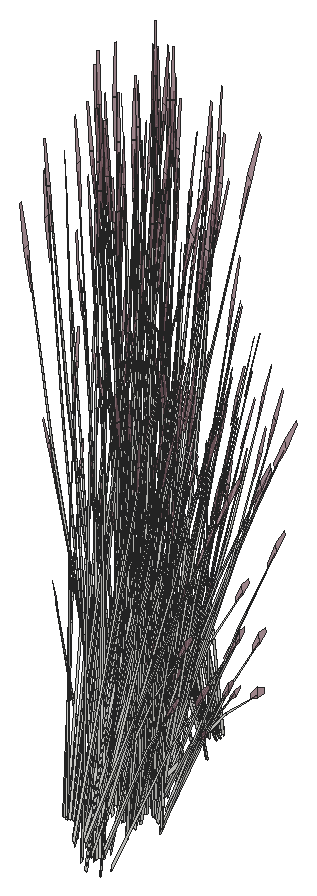
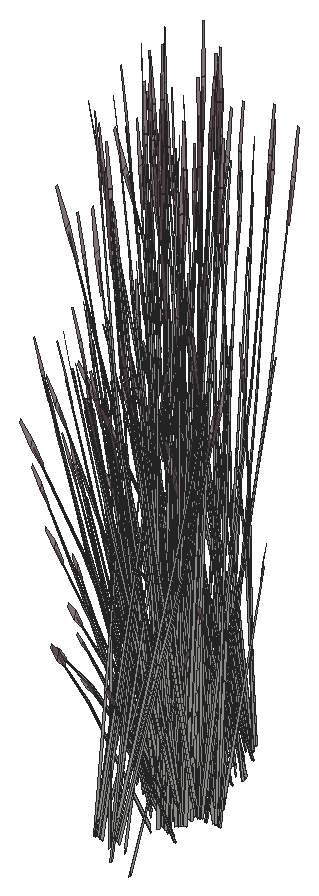
# SketchUp Ruby script. Lengths in inches.
U = 1.inch
M = Sketchup.active_model
def pt(a) = Geom::Point3d.new(a.map { |v| v * U })
def face(e, loops, mat)
  f = e.add_face(loops[0].map { |a| pt(a) })
  loops[1..].each { |l| e.add_face(l.map { |a| pt(a) }).erase! }
  f.material = f.back_material = mat if mat
  f
end
# faces: each face lists its corners as indices into pts; further lists are holes
def faces(e, pts, list, mat = nil) = list.each { |f| face(e, (f[0].is_a?(Array) ? f : [f]).map { |l| l.map { |i| pts[i] } }, mat) }
# xy, xz, yz: faces in a plane at the given z, y or x. An outline is a flat list of corners, or four numbers for a rectangle; further outlines are holes
def ring(l) = l.size == 4 ? [[l[0], l[1]], [l[2], l[1]], [l[2], l[3]], [l[0], l[3]]] : l.each_slice(2).to_a
def flat(e, list, mat, &to3) = list.each { |f| face(e, (f[0].is_a?(Array) ? f : [f]).map { |l| ring(l).map { |u, v| to3.(u, v) } }, mat) }
def xy(e, z, list, mat = nil) = flat(e, list, mat) { |x, y| [x, y, z] }
def xz(e, y, list, mat = nil) = flat(e, list, mat) { |x, z| [x, y, z] }
def yz(e, x, list, mat = nil) = flat(e, list, mat) { |y, z| [x, y, z] }
def lines(e, pts, list) = list.each { |a, b| e.add_line(pt(pts[a]), pt(pts[b])) }
# prism: a flat outline (further loops are holes) pulled along v
def prism(e, loops, v, mat = nil)
  f = face(e, loops, mat); d = Geom::Vector3d.new(v.map { |x| x * U })
  f.pushpull(f.normal.samedirection?(d) ? d.length : -d.length)
end
def box(e, o, s, mat = nil) = prism(e, [[o, [o[0] + s[0], o[1], o[2]], [o[0] + s[0], o[1] + s[1], o[2]], [o[0], o[1] + s[1], o[2]]]], [0, 0, s[2]], mat)
def at(x, y, z, deg = 0) = Geom::Transformation.translation(pt([x, y, z])) * Geom::Transformation.rotation(ORIGIN, Z_AXIS, deg.degrees)
def axes(o, x, y, z) = Geom::Transformation.new([*x, 0, *y, 0, *z, 0, *pt(o).to_a, 1])
def part(name) = M.definitions.add(name)
# library, detail: a bought-in or finely detailed component or shape, given as its bounding box
def library(name, o, s) = part(name).tap { |d| box(d.entities, o, s) }
def detail(e, o, s) = box(e.add_group.entities, o, s)
def put(e, d, t, mat = nil) = e.add_instance(d, t).tap { |i| i.material = mat if mat }
def group(e, t, mat = nil) = e.add_group.tap { |g| g.transformation = t; g.material = mat if mat }.entities
root = M.entities
M.materials.add("LightPink_Translucent").color = [144, 107, 117]
M.materials["LightPink_Translucent"].alpha = 0.75
c1 = part("blade")
p = [[2.15,0.21,22],[0,0.17,0],[0.09,0.45,0],[2.18,0.31,22],[2.29,0.31,22],[0.38,0.45,0],
  [2.48,0.24,33],[2.49,0.24,33],[2.48,0.22,33]]
faces(c1.entities,p,[[0,1,2,3],[4,5,2,3],[6,3,4,7],[8,0,3,6]])
c2 = part("seeds")
p = [[0.3,-0.1,1.38],[-0.01,-0.03,1.59],[-0.01,-0.03,0.03],[0.14,-0.07,-0.07],[0.29,-0.03,3],[0.15,0.01,3.11]]
faces(c2.entities,p,[[0,1,2,3],[1,0,4,5]],"LightPink_Translucent")
c3 = part("blade with seeds")
put(c3.entities,c1,at(0,0,0))
put(c3.entities,c2,axes([2.4,0.25,30.99],[1.5799,-0.05474,1.17369],[-0.12525,1.92788,0.29478],[-0.07173,-0.02425,1.56792]))
put(root,c3,axes([410.79,313.69,-7.3],[-0.07899,-0.43781,0.32977],[0.45153,-0.11561,-0.42575],[0.12128,0.12546,0.81462]))
put(root,c3,axes([410.94,313.53,-9.83],[0.64025,0.17667,0.2864],[-0.16018,0.63149,-0.33981],[-0.10597,0.07904,1.53541]))
put(root,c3,axes([410.89,313.96,-10.12],[-0.47863,0.27177,-0.46235],[-0.28609,-0.48733,0],[-0.10901,0.0619,1.46668]))
put(root,c3,axes([412.48,312.35,-10.12],[0,0.54355,-0.46235],[-0.57217,0,0],[0,0.1238,1.46668]))
put(root,c3,axes([411.05,312.41,-8.39],[-0.18996,-0.09365,1.59586],[0.39312,-0.39287,0.12904],[0.24502,0.17723,0.68222]))
put(root,c3,axes([411.09,311.18,-7.83],[-0.44191,-0.28242,1.28769],[0.46662,-0.43971,0.5556],[0.14258,0.26499,1.24467]))
put(root,c3,axes([407.39,319.84,-10.05],[-0.21003,-0.55738,-0.65031],[0.60499,-0.20074,-0.17068],[-0.02321,-0.18874,1.43544]))
put(root,c3,axes([410.2,318.14,-10.61],[-0.07655,-0.04282,1.6421],[-0.19662,-0.47839,-0.25086],[0.13264,-0.12982,0.2797]))
put(root,c3,axes([411.76,313.47,-9.42],[-0.28795,-0.15629,1.06958],[0.37181,-0.1588,0.78586],[0.10029,0.13452,0.23558]))
put(root,c3,axes([410.75,313.92,-7.3125],[0.30474,-0.46525,-0.11324],[0.44133,0.26804,-0.62851],[0.15341,0.13145,0.95501]))
put(root,c3,axes([408.62,318.25,-7.3],[-0.15418,0.41799,0.32977],[-0.44981,-0.12192,-0.42575],[-0.04124,-0.16829,0.81462]))
put(root,c3,axes([409.77,318.42,-7.59],[0.36417,0.37086,0.447],[-0.38674,0.31985,0.36857],[0.06718,-0.174,0.92496]))
put(root,c3,axes([409.9,318.46,-7.6],[0.42027,0.02533,0.05988],[-0.01152,0.38243,0.47138],[0.04398,-0.14649,0.71878]))
put(root,c3,axes([408.74,313.29,-7.3],[0.34603,-0.28618,0.32977],[0.32756,0.32677,-0.42575],[-0.04984,0.16603,0.81462]))
put(root,c3,axes([411.33,313.87,-9.79],[0.31974,0.54466,0],[-0.53494,0.30375,-0.48057],[-0.12184,0.06918,1.52448]))
put(root,c3,axes([410.35,314.31,-7.62],[0.00151,-0.06581,1.65179],[0.43826,-0.29033,-0.15608],[0.15223,0.10363,0.29231]))
put(root,c3,axes([409.59,318.72,-7.3],[-0.34603,0.28618,0.32977],[-0.32756,-0.32677,-0.42575],[0.04984,-0.16603,0.81462]))
put(root,c3,axes([411.84,314.05,-10.61],[0.03726,-0.07847,1.6421],[0.46909,-0.23111,-0.25086],[0.14221,0.11962,0.2797]))
put(root,c3,axes([411.06,311.72,-9.35],[-0.01397,-0.51177,1.31553],[0.63227,0.13266,0.557],[-0.14954,0.28003,1.24175]))
put(root,c3,axes([411.22,312.27,-10.05],[0.18752,0.49766,-0.6445],[-0.54017,0.17923,-0.16915],[0.02073,0.16852,1.42262]))
put(root,c3,axes([408.42,313.55,-7.6],[-0.42027,-0.02533,0.05988],[0.01152,-0.38243,0.47138],[-0.04398,0.14649,0.71878]))
put(root,c3,axes([410.2,319.49,-7.36],[0.26714,-0.42887,-0.66157],[0.46811,0.30479,0.07984],[0.1595,-0.15539,0.93586]))
put(root,c3,axes([408.56,313.59,-7.59],[-0.36417,-0.37086,0.447],[0.38674,-0.31985,0.36857],[-0.06718,0.174,0.92496]))
put(root,c3,axes([407.31,318.24,-9.79],[-0.31974,-0.54466,0],[0.53494,-0.30375,-0.48057],[0.12184,-0.06918,1.52448]))
put(root,c3,axes([410.19,319.29,-7.64],[-0.13138,-0.49631,-0.47583],[0.49754,-0.08682,-0.36857],[0.14258,-0.13331,0.91046]))
put(root,c3,axes([411.11,313.69,-7.64],[0.50465,-0.12921,-0.47583],[0.08828,0.48932,-0.36857],[0.13555,0.14022,0.91046]))
put(root,c3,axes([408.01,317.58,-10.02],[-0.35341,0.31182,-0.03625],[-0.32382,-0.34152,-0.16435],[-0.0228,-0.09677,0.54209]))
put(root,c3,axes([409.71,313.76,-7.3],[0.15418,-0.41799,0.32977],[0.44981,0.12192,-0.42575],[0.04124,0.16829,0.81462]))
put(root,c3,axes([410.42,319.64,-7.3125],[-0.47307,-0.29971,-0.11324],[0.27254,-0.43404,-0.62851],[0.13365,-0.15087,0.95501]))
put(root,c3,axes([411.8,314.1875,-9.52],[-0.32795,-0.01705,0.97832],[0.21658,-0.36206,0.54015],[0.12956,0.12863,0.76741]))
put(root,c3,axes([410.86,314.09,-7.6],[-0.23243,0.34529,0.05988],[-0.331,-0.20103,0.47138],[0.10701,0.1107,0.71878]))
put(root,c3,axes([410.3125,315.25,-6.74],[0.35341,-0.31182,-0.06041],[0.32382,0.34152,-0.27392],[0.0228,0.09677,0.90349]))
put(root,c3,axes([410.96,313.99,-7.59],[-0.50866,0.12474,0.447],[-0.08828,-0.48932,0.36857],[0.11963,0.14421,0.92496]))
put(root,c3,axes([406.16,319.77,-10.12],[0,-0.54355,-0.46235],[0.57217,0,0],[0,-0.1238,1.46668]))
put(root,c3,axes([407.74,318.16,-10.12],[0.47863,-0.27177,-0.46235],[0.28609,0.48733,0],[0.10901,-0.0619,1.46668]))
put(root,c3,axes([410.59,319.1,-9.59],[-0.1827,-0.0161,1.33163],[-0.18717,-0.43188,-0.28638],[0.22444,-0.12218,0.56934]))
put(root,c3,axes([411.58,319.51,-7.62],[-0.0668,-0.00413,1.65179],[-0.27738,-0.44233,-0.15608],[0.11139,-0.14544,0.29231]))
put(root,c3,axes([410.73,313.31,-9.59],[0.00902,-0.18018,1.33163],[0.43127,-0.20126,-0.28638],[0.13313,0.21566,0.56934]))
put(root,c3,axes([408.3125,319.27,-10.08],[0.34446,-0.40855,-0.58063],[0.42791,0.37046,-0.15239],[0.13803,-0.10191,1.28164]))
put(root,c3,axes([410.8,318.3,-9.42],[-0.17034,0.27669,1.06958],[-0.14642,-0.37174,0.78586],[0.14069,-0.09315,0.23558]))
put(root,c3,axes([409.57,314.14,-7.6],[-0.37684,0.18473,0.05988],[-0.18445,-0.33686,0.47138],[0.03639,0.14849,0.71878]))
put(root,c3,axes([408.56,313.7,-7.78],[-0.34603,0.28618,-0.32977],[-0.32756,-0.32677,0.42575],[-0.04984,0.16603,0.81462]))
put(root,c3,axes([408.52,313.37,-6.97],[0.56206,0.02693,-0.12569],[-0.01536,0.50991,-0.69765],[-0.03904,0.19638,1.06006]))
put(root,c3,axes([409.56,313.9375,-7.3125],[0.50045,-0.25306,-0.11324],[0.24593,0.44915,-0.62851],[0.06603,0.18927,0.95501]))
put(root,c3,axes([409.7,314.11,-7.28],[-0.50393,-0.1421,0.49617],[0.17232,-0.46717,0.40911],[0.03028,0.18372,1.0267]))
put(root,c3,axes([410.55,319.34,-7.78],[0.44516,-0.07768,-0.32977],[0.11755,0.44407,0.42575],[0.12757,-0.11927,0.81462]))
put(root,c3,axes([408.78,314.81,-9.42],[-0.01324,-0.32319,1.06958],[0.33072,0.23052,0.78586],[-0.06504,0.15405,0.23558]))
put(root,c3,axes([407.71,319.99,-9.94],[0.24813,-0.48978,-0.41661],[0.51557,0.23571,0.2005],[0,-0.1129,1.33761]))
put(root,c3,axes([407.9375,319.74,-9.52],[-0.05959,-0.62022,-0.27094],[0.62068,-0.0375,-0.46562],[0.1093,-0.08261,1.4872]))
put(root,c3,axes([409.65,314.04,-10.61],[0.08277,-0.02958,1.6421],[0.49786,0.16279,-0.25086],[0.01456,0.18348,0.2797]))
put(root,c3,axes([406.4,319.78,-10.11],[0.35699,-0.33913,-0.28847],[0.35699,0.33913,0.28847],[0,-0.10923,1.29413]))
put(root,c3,axes([410.1875,319.6,-7.3],[-0.44516,0.07768,0.32977],[-0.11755,-0.44407,-0.42575],[0.12757,-0.11927,0.81462]))
put(root,c3,axes([407.65,320.39,-9.52],[-0.57594,-0.25935,-0.27094],[0.27732,-0.5474,-0.46562],[-0.0181,-0.1344,1.4872]))
put(root,c3,axes([408.9,313.5625,-7.34],[0.3661,0.36521,-0.52818],[-0.38674,0.31985,-0.40911],[-0.0557,0.18556,1.01061]))
put(root,c3,axes([408.5,314.11,-9.37],[0.46459,-0.09625,0.0606],[0.10681,0.38778,-0.80367],[-0.02945,0.1963,0.72038]))
put(root,c3,axes([409.99,313.92,-7.64],[0.50273,0.13626,-0.47583],[-0.17232,0.46717,-0.36857],[0.0461,0.18809,0.91046]))
put(root,c3,axes([410.27,312.95,-8.39],[-0.1169,-0.17452,1.59586],[0.54019,-0.14692,0.12904],[0.12209,0.27397,0.68222]))
put(root,c3,axes([407.86,318.37,-10.11],[0.47712,0.13449,-0.28847],[-0.12013,0.47362,0.28847],[0.09619,-0.05462,1.29413]))
put(root,c3,axes([409.76,314.2,-7.78],[-0.15418,0.41799,-0.32977],[-0.44981,-0.12192,0.42575],[0.04124,0.16829,0.81462]))
put(root,c3,axes([408.79,313.4,-7.03],[-0.01331,0.50278,-0.73435],[-0.56035,-0.03377,0.08862],[-0.05914,0.213,1.03881]))
put(root,c3,axes([407.32,314.72,-7.62],[0.05802,-0.03282,1.65179],[0.47954,0.21828,-0.15608],[-0.01127,0.18175,0.29231]))
put(root,c3,axes([410.59,319.53,-7.6],[0.35109,0.22859,0.05988],[-0.2044,0.32553,0.47138],[0.11256,-0.10524,0.71878]))
put(root,c3,axes([410.49,319.4375,-7.59],[0.12683,0.50025,0.447],[-0.49754,0.08682,0.36857],[0.14663,-0.11765,0.92496]))
put(root,c3,axes([411.84,320.04,-7.61],[0.07097,-0.08279,1.62908],[-0.09083,-0.50786,-0.25764],[0.17806,-0.09629,0.13065]))
put(root,c3,axes([409.32,313.04,-8.39],[-0.01252,-0.20862,1.59586],[0.54251,0.1384,0.12904],[-0.03356,0.2973,0.68222]))
put(root,c3,axes([409.8,313.83,-7.36],[0.24409,0.44196,-0.66157],[-0.50245,0.2463,0.07984],[0.05708,0.21354,0.93586]))
put(root,c3,axes([408.02,320.23,-9.73],[0.57623,0.26344,0.22409],[-0.27732,0.5474,0.46562],[0,-0.12618,1.49497]))
put(root,c3,axes([408.39,314.52,-9.59],[0.16138,-0.08575,1.33163],[0.39845,0.25854,-0.28638],[-0.1186,0.22371,0.56934]))
put(root,c3,axes([409.4375,314.94,-7.61],[0.06483,0.08753,1.62908],[0.52315,0.03439,-0.25764],[0.05261,0.19303,0.13065]))
put(root,c3,axes([407.83,319.86,-9.47],[-0.55535,0.03355,0.41661],[-0.05022,-0.55698,-0.2005],[0.09942,-0.05645,1.33761]))
put(root,c3,axes([406.4,320.27,-9.69],[0,0.54355,0.46235],[-0.57217,0,0],[0,-0.1238,1.46668]))
put(root,c3,axes([410.4375,320.8125,-7.3125],[-0.25732,-0.49218,-0.11324],[0.45669,-0.24187,-0.62851],[0.19245,-0.06494,0.95501]))
put(root,c3,axes([410.42,320.39,-7.64],[0.13855,-0.49442,-0.47583],[0.47502,0.16947,-0.36857],[0.19125,-0.04534,0.91046]))
put(root,c3,axes([409.67,318.38,-9.79],[0.31974,-0.54466,0],[0.53494,0.30375,-0.48057],[0.12184,0.06918,1.52448]))
put(root,c3,axes([407.81,320.06,-9.8],[0.22235,0.6078,0.42607],[-0.63531,0.21135,0.16719],[0.00776,-0.11168,1.47927]))
put(root,c3,axes([410.92,320.53,-10.15],[-0.32938,0.06523,1.31842],[-0.05243,-0.51922,0.07547],[0.2307,-0.07859,0.75023]))
put(root,c3,axes([411.52,320.07,-9.89],[-0.31706,-0.34757,-0.06041],[0.34725,-0.31847,-0.27392],[0.09839,-0.02242,0.90349]))
put(root,c3,axes([408.6,314.1,-8.87],[0.01124,-0.2806,1.43727],[0.50537,0.14821,0.19862],[-0.04379,0.29905,0.67868]))
put(root,c3,axes([407.7,320.54,-9.47],[-0.24813,0.48978,0.41661],[-0.51557,-0.23571,-0.2005],[0,-0.1129,1.33761]))
put(root,c3,axes([408.61,320.12,-9.95],[0,-0.62892,0],[0.63949,0,0],[0,0,1.6711]))
put(root,c3,axes([409.39,318.66,-9.69],[-0.47863,-0.27177,0.46235],[0.28609,-0.48733,0],[0.10901,0.0619,1.46668]))
put(root,c3,axes([410.33,320.57,-7.36],[0.44939,-0.24006,-0.66157],[0.25044,0.49415,0.07984],[0.21713,-0.05613,0.93586]))
put(root,c3,axes([408.3125,319.72,-9.8],[-0.42403,0.49328,0.42607],[-0.50377,-0.43543,0.16719],[0.10223,-0.04923,1.47927]))
put(root,c3,axes([408.77,320.6,-9.86],[-0.47569,-0.46784,-0.05709],[0.47598,-0.46812,0],[-0.01661,-0.01634,1.63492]))
put(root,c3,axes([407.58,318.91,-9.7],[-0.14774,0.54019,0.16428],[-0.54062,-0.15287,0.32672],[0.09339,-0.00263,1.49371]))
put(root,c3,axes([410.26,320.67,-7.3],[-0.42502,-0.15163,0.32977],[0.12396,-0.44238,-0.42575],[0.17112,-0.04056,0.81462]))
put(root,c3,axes([407.35,319.34,-10.52],[-0.50338,0.21762,1.20058],[-0.16022,-0.62439,0.4665],[0.30911,0.01039,1.36553]))
put(root,c3,axes([408.7,319.51,-9.5625],[0.09866,-0.48509,0.13483],[0.48202,0.0842,-0.38503],[0.08772,0.04981,1.18024]))
put(root,c3,axes([407.87,320.66,-9.8],[0.64638,0.11452,0.42607],[-0.13155,0.64678,0.16719],[-0.09446,-0.06245,1.47927]))
put(root,c3,axes([411.28,320.19,-10.61],[-0.02673,-0.08252,1.6421],[0.18538,-0.48271,-0.25086],[0.187,-0.00694,0.2797]))
put(root,c3,axes([408.5,319.64,-9.47],[-0.30722,-0.45622,0.41661],[0.46535,-0.32126,-0.2005],[0.09942,0.05645,1.33761]))
put(root,c3,axes([407.52,321.69,-9.7],[0.54955,-0.14427,0.16428],[0.1357,0.53689,0.32672],[-0.04901,-0.07823,1.49371]))
put(root,c3,axes([408.66,319.67,-9.52],[0.51635,-0.36087,-0.27094],[0.34336,0.5099,-0.46562],[0.1274,0.05178,1.4872]))
put(root,c3,axes([410.71,320.62,-7.78],[0.42502,0.15163,-0.32977],[-0.12396,0.44238,0.42575],[0.17112,-0.04056,0.81462]))
put(root,c3,axes([409.96,318.71,-10.12],[0.47863,0.27177,-0.46235],[-0.28609,0.48733,0],[0.10901,0.0619,1.46668]))
put(root,c3,axes([409.05,320.26,-9.95],[0.57217,0,0],[0,0.56272,0],[0,0,1.66132]))
put(root,c3,axes([409.21,318.9375,-9.7],[-0.54955,0.14427,0.16428],[-0.1357,-0.53689,0.32672],[0.04901,0.07823,1.49371]))
put(root,c3,axes([409.55,320.07,-8.39],[-0.21212,0.01231,1.59586],[0.14072,-0.53355,0.12904],[0.3023,0.033,0.68222]))
put(root,c3,axes([409.82,318.91,-10.11],[0.12013,0.47362,-0.28847],[-0.47712,0.13449,0.28847],[0.09619,0.05462,1.29413]))
put(root,c3,axes([410.65,320.8,-7.6],[0.18783,0.37061,0.05988],[-0.34252,0.1814,0.47138],[0.15099,-0.03579,0.71878]))
put(root,c3,axes([408.86,319.97,-9.78],[-0.64638,-0.11452,0.45814],[0.13155,-0.64678,0.17978],[0.09446,0.06245,1.59061]))
put(root,c3,axes([410.61,320.67,-7.59],[-0.14449,0.4956,0.447],[-0.47502,-0.16947,0.36857],[0.1868,-0.02978,0.92496]))
put(root,c3,axes([408.35,321.57,-9.95],[-0.16686,-0.46861,0],[0.47648,-0.16411,0],[0,0,1.4375]))
put(root,c3,axes([408.97,321.5,-9.97],[0.53691,-0.18442,-0.17877],[0.18866,0.53125,0.00007],[0.05927,-0.02038,1.61933]))
put(root,c3,axes([409.16,321.72,-9.7],[0.14774,-0.54019,0.16428],[0.54062,0.15287,0.32672],[-0.09339,0.00263,1.49371]))
put(root,c3,axes([409.04,320.5,-9.9375],[0.35699,0.35109,0],[-0.35699,0.35109,0],[0,0,1.57621]))
put(root,c3,axes([410,320.34,-9.7],[-0.40181,-0.39593,0.16428],[0.40492,-0.38402,0.32672],[-0.04438,0.08086,1.49371]))
put(root,c3,axes([409.26,319.75,-10.08],[0.53199,0.08911,-0.58063],[-0.11226,0.54969,-0.15239],[0.15876,0.06661,1.28164]))
put(root,c3,axes([411.61,320.71,-9.42],[-0.31598,0.08973,1.06958],[0.14873,-0.37085,0.78586],[0.16763,0.02538,0.23558]))
put(root,c3,axes([408.23,321.78,-9.95],[-0.51557,-0.24403,0],[0.24813,-0.50705,0],[0,0,1.51513]))
put(root,c3,axes([409.03,320.09,-9.47],[0.24813,-0.48978,0.41661],[0.51557,0.23571,-0.2005],[0,0.1129,1.33761]))
put(root,c3,axes([411.46,322.28,-7.62],[-0.04624,-0.04758,1.65179],[0.10116,-0.51007,-0.15608],[0.18215,-0.03259,0.29231]))
put(root,c3,axes([408.9375,320.37,-9.87],[0,0.62861,-0.05249],[-0.63949,0,0],[0,0.01975,1.67027]))
put(root,c3,axes([408.98,319.92,-9.94],[0.30722,0.45622,-0.41661],[-0.46535,0.32126,0.2005],[0.09942,0.05645,1.33761]))
put(root,c3,axes([411.06,321.85,-8.34],[-0.09788,-0.45691,-0.03251],[0.46264,-0.10504,-0.14742],[0.09661,0.02897,0.48626]))
put(root,c3,axes([409.86,321.84,-7.3125],[0.02738,-0.55277,-0.11324],[0.51847,0.01511,-0.62851],[0.19968,0.0384,0.95501]))
put(root,c3,axes([410.33,320.36,-9.69],[0,-0.54355,0.46235],[0.57217,0,0],[0,0.1238,1.46668]))
put(root,c3,axes([408.9,320.77,-9.47],[0.55535,-0.03355,0.41661],[0.05022,0.55698,-0.2005],[-0.09942,0.05645,1.33761]))
put(root,c3,axes([409.25,320.2,-9.5625],[0.47648,-0.15851,0.13483],[0.16686,0.45265,-0.38503],[0,0.09962,1.18024]))
put(root,c3,axes([409.78,321.62,-7.3],[-0.29098,-0.34031,0.32977],[0.33226,-0.32215,-0.42575],[0.16881,0.04902,0.81462]))
put(root,c3,axes([411.02,321.3,-9.59],[-0.12317,-0.13368,1.33163],[0.16025,-0.44223,-0.28638],[0.24919,0.05991,0.56934]))
put(root,c3,axes([408.82,321.79,-9.95],[0.51557,0.24403,0],[-0.24813,0.50705,0],[0,0,1.62917]))
put(root,c3,axes([410.3125,321.5,-7.61],[0.10971,-0.00919,1.62908],[0.30091,-0.42228,-0.25764],[0.19514,0.05574,0.13065]))
put(root,c3,axes([409.02,322.33,-9.96],[-0.31576,-0.54657,-0.04789],[0.53494,-0.30375,0.48057],[-0.13182,0.05204,1.52373]))
put(root,c3,axes([408.91,321.01,-9.5625],[0.37783,0.32657,0.13483],[-0.31516,0.36844,-0.38503],[-0.08772,0.04981,1.18024]))
put(root,c3,axes([409.89,321.57,-7.36],[0.51122,0.01309,-0.66157],[-0.03434,0.5511,0.07984],[0.21658,0.05816,0.93586]))
put(root,c3,axes([409.3125,322.01,-9.69],[0.47863,-0.27177,0.46235],[0.28609,0.48733,0],[-0.10901,0.0619,1.46668]))
put(root,c3,axes([408.63,321.58,-9.87],[0.22235,0.62444,-0.05599],[-0.63531,0.21881,0],[0.00776,0.02181,1.60327]))
put(root,c3,axes([408.875,322.26,-10.11],[-0.47712,-0.13449,-0.28847],[0.12013,-0.47362,0.28847],[-0.09619,0.05462,1.29413]))
put(root,c3,axes([410.72,320.45,-9.79],[0.63949,0,0],[0,0.60749,-0.48057],[0,0.13836,1.52448]))
put(root,c3,axes([410.47,320.76,-9.95],[-0.63917,-0.00435,-0.04634],[0,-0.60749,0.46507],[-0.02009,0.13829,1.47457]))
put(root,c3,axes([409.08,320.24,-9.52],[0.57594,0.25935,-0.27094],[-0.27732,0.5474,-0.46562],[0.0181,0.1344,1.4872]))
put(root,c3,axes([410.19,321.8,-7.78],[0.29098,0.34031,-0.32977],[-0.33226,0.32215,0.42575],[0.16881,0.04902,0.81462]))
put(root,c3,axes([410.33,320.85,-10.11],[-0.35699,0.33913,-0.28847],[-0.35699,-0.33913,0.28847],[0,0.10923,1.29413]))
put(root,c3,axes([408.79,320.89,-9.52],[0.05959,0.62022,-0.27094],[-0.62068,0.0375,-0.46562],[-0.1093,0.08261,1.4872]))
put(root,c3,axes([410.04,321.93,-7.6],[-0.02575,0.41332,0.05988],[-0.38885,-0.01133,0.47138],[0.14895,0.04325,0.71878]))
put(root,c3,axes([409.02,320.64,-9.94],[-0.24813,0.48978,-0.41661],[-0.51557,-0.23571,0.2005],[0,0.1129,1.33761]))
put(root,c3,axes([410.08,321.8,-7.59],[-0.37709,0.35815,0.447],[-0.32522,-0.38035,0.36857],[0.17692,0.06607,0.92496]))
put(root,c3,axes([408.88,322.21,-7.3],[-0.07899,-0.43781,0.32977],[0.45153,-0.11561,-0.42575],[0.12128,0.12546,0.81462]))
put(root,c3,axes([409.03,322.05,-9.83],[0.64025,0.17667,0.2864],[-0.16018,0.63149,-0.33981],[-0.10597,0.07904,1.53541]))
put(root,c3,axes([408.99,322.47,-10.12],[-0.47863,0.27177,-0.46235],[-0.28609,-0.48733,0],[-0.10901,0.0619,1.46668]))
put(root,c3,axes([410.58,320.86,-10.12],[0,0.54355,-0.46235],[-0.57217,0,0],[0,0.1238,1.46668]))
put(root,c3,axes([409.15,320.93,-8.39],[-0.18996,-0.09365,1.59586],[0.39312,-0.39287,0.12904],[0.24502,0.17723,0.68222]))
put(root,c3,axes([409.19,319.69,-7.83],[-0.44191,-0.28242,1.28769],[0.46662,-0.43971,0.5556],[0.14258,0.26499,1.24467]))
put(root,c3,axes([409.85,321.99,-9.42],[-0.28795,-0.15629,1.06958],[0.37181,-0.1588,0.78586],[0.10029,0.13452,0.23558]))
put(root,c3,axes([408.84,322.4375,-7.3125],[0.30474,-0.46525,-0.11324],[0.44133,0.26804,-0.62851],[0.15341,0.13145,0.95501]))
put(root,c3,axes([406.83,321.81,-7.3],[0.34603,-0.28618,0.32977],[0.32756,0.32677,-0.42575],[-0.04984,0.16603,0.81462]))
put(root,c3,axes([408.64,328.7,-9.59],[-0.14537,0.11002,1.33163],[-0.43536,-0.19256,-0.28638],[0.0807,-0.23948,0.56934]))
put(root,c3,axes([409.42,322.39,-9.79],[0.31974,0.54466,0],[-0.53494,0.30375,-0.48057],[-0.12184,0.06918,1.52448]))
put(root,c3,axes([407.97,329.08,-7.36],[-0.24409,-0.44196,-0.66157],[0.50245,-0.2463,0.07984],[-0.05708,-0.21354,0.93586]))
put(root,c3,axes([408.44,322.82,-7.62],[0.00151,-0.06581,1.65179],[0.43826,-0.29033,-0.15608],[0.15223,0.10363,0.29231]))
put(root,c3,axes([409.93,322.57,-10.61],[0.03726,-0.07847,1.6421],[0.46909,-0.23111,-0.25086],[0.14221,0.11962,0.2797]))
put(root,c3,axes([409.15,320.23,-9.35],[-0.01397,-0.51177,1.31553],[0.63227,0.13266,0.557],[-0.14954,0.28003,1.24175]))
put(root,c3,axes([409.3125,320.79,-10.05],[0.18752,0.49766,-0.6445],[-0.54017,0.17923,-0.16915],[0.02073,0.16852,1.42262]))
put(root,c3,axes([409.2,322.21,-7.64],[0.50465,-0.12921,-0.47583],[0.08828,0.48932,-0.36857],[0.13555,0.14022,0.91046]))
put(root,c3,axes([407.8,322.28,-7.3],[0.15418,-0.41799,0.32977],[0.44981,0.12192,-0.42575],[0.04124,0.16829,0.81462]))
put(root,c3,axes([407.55,328.1,-10.61],[-0.08578,0.01958,1.6421],[-0.47437,-0.22044,-0.25086],[0.00796,-0.18387,0.2797]))
put(root,c3,axes([409.9,322.7,-9.52],[-0.32795,-0.01705,0.97832],[0.21658,-0.36206,0.54015],[0.12956,0.12863,0.76741]))
put(root,c3,axes([408.99,329.51,-7.36],[0.01331,-0.50278,-0.66157],[0.56035,0.03377,0.07984],[0.05914,-0.213,0.93586]))
put(root,c3,axes([408.95,322.61,-7.6],[-0.23243,0.34529,0.05988],[-0.331,-0.20103,0.47138],[0.10701,0.1107,0.71878]))
put(root,c3,axes([409.77,328.73,-7.61],[-0.00494,-0.10818,1.62908],[-0.41695,-0.31265,-0.25764],[0.06446,-0.18952,0.13065]))
put(root,c3,axes([408.02,328.71,-7.78],[0.15418,-0.41799,-0.32977],[0.44981,0.12192,0.42575],[-0.04124,-0.16829,0.81462]))
put(root,c3,axes([408.36,329.26,-8.39],[-0.09522,0.18683,1.59586],[-0.39947,-0.38663,0.12904],[0.18021,-0.24097,0.68222]))
put(root,c3,axes([409.66,328.34,-7.62],[-0.05194,0.04152,1.65179],[-0.50886,-0.14007,-0.15608],[-0.01842,-0.18118,0.29231]))
put(root,c3,axes([408.41,323.77,-6.74],[0.35341,-0.31182,-0.06041],[0.32382,0.34152,-0.27392],[0.0228,0.09677,0.90349]))
put(root,c3,axes([409.05,322.51,-7.59],[-0.50866,0.12474,0.447],[-0.08828,-0.48932,0.36857],[0.11963,0.14421,0.92496]))
put(root,c3,axes([407.79,328.99,-7.64],[-0.50273,-0.13626,-0.47583],[0.17232,-0.46717,-0.36857],[-0.0461,-0.18809,0.91046]))
put(root,c3,axes([408.1,327.82,-9.42],[0.06561,0.31695,1.06958],[-0.36394,-0.17555,0.78586],[0.03916,-0.16229,0.23558]))
put(root,c3,axes([408.875,329.35,-7.64],[-0.3661,-0.36521,-0.47583],[0.38674,-0.31985,-0.36857],[0.0557,-0.18556,0.91046]))
put(root,c3,axes([408.83,321.83,-9.59],[0.00902,-0.18018,1.33163],[0.43127,-0.20126,-0.28638],[0.13313,0.21566,0.56934]))
put(root,c3,axes([407.66,322.66,-7.6],[-0.37684,0.18473,0.05988],[-0.18445,-0.33686,0.47138],[0.03639,0.14849,0.71878]))
put(root,c3,axes([406.61,321.89,-6.97],[0.56206,0.02693,-0.12569],[-0.01536,0.50991,-0.69765],[-0.03904,0.19638,1.06006]))
put(root,c3,axes([407.65,322.46,-7.3125],[0.50045,-0.25306,-0.11324],[0.24593,0.44915,-0.62851],[0.06603,0.18927,0.95501]))
put(root,c3,axes([407.8,322.625,-7.28],[-0.50393,-0.1421,0.49617],[0.17232,-0.46717,0.40911],[0.03028,0.18372,1.0267]))
put(root,c3,axes([408.08,328.8,-7.59],[0.50393,0.1421,0.447],[-0.17232,0.46717,0.36857],[-0.03028,-0.18372,0.92496]))
put(root,c3,axes([408.22,328.97,-7.3125],[-0.50045,0.25306,-0.11324],[-0.24593,-0.44915,-0.62851],[-0.06603,-0.18927,0.95501]))
put(root,c3,axes([409.26,329.54,-7.3125],[-0.56206,-0.02693,-0.11324],[0.01536,-0.50991,-0.62851],[0.03904,-0.19638,0.95501]))
put(root,c3,axes([409.22,329.21,-7.78],[0.34603,-0.28618,-0.32977],[0.32756,0.32677,0.42575],[0.04984,-0.16603,0.81462]))
put(root,c3,axes([407.74,322.56,-10.61],[0.08277,-0.02958,1.6421],[0.49786,0.16279,-0.25086],[0.01456,0.18348,0.2797]))
put(root,c3,axes([408.21,328.77,-7.6],[0.37684,-0.18473,0.05988],[0.18445,0.33686,0.47138],[-0.03639,-0.14849,0.71878]))
